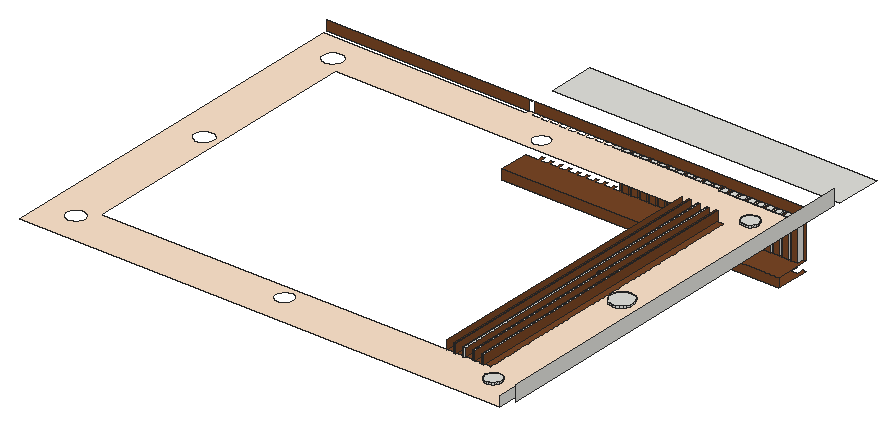
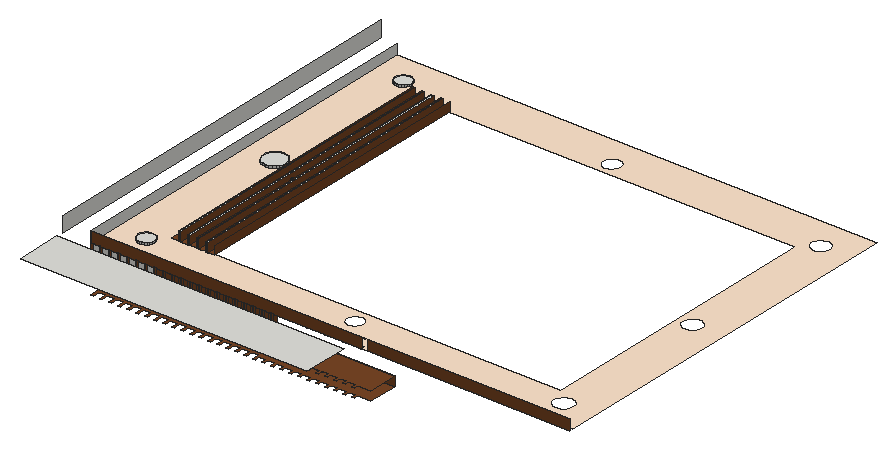
# SketchUp Ruby script. Lengths in inches.
U = 1.inch
M = Sketchup.active_model
def pt(a) = Geom::Point3d.new(a.map { |v| v * U })
def face(e, loops, mat)
  f = e.add_face(loops[0].map { |a| pt(a) })
  loops[1..].each { |l| e.add_face(l.map { |a| pt(a) }).erase! }
  f.material = f.back_material = mat if mat
  f
end
# faces: each face lists its corners as indices into pts; further lists are holes
def faces(e, pts, list, mat = nil) = list.each { |f| face(e, (f[0].is_a?(Array) ? f : [f]).map { |l| l.map { |i| pts[i] } }, mat) }
# xy, xz, yz: faces in a plane at the given z, y or x. An outline is a flat list of corners, or four numbers for a rectangle; further outlines are holes
def ring(l) = l.size == 4 ? [[l[0], l[1]], [l[2], l[1]], [l[2], l[3]], [l[0], l[3]]] : l.each_slice(2).to_a
def flat(e, list, mat, &to3) = list.each { |f| face(e, (f[0].is_a?(Array) ? f : [f]).map { |l| ring(l).map { |u, v| to3.(u, v) } }, mat) }
def xy(e, z, list, mat = nil) = flat(e, list, mat) { |x, y| [x, y, z] }
def xz(e, y, list, mat = nil) = flat(e, list, mat) { |x, z| [x, y, z] }
def yz(e, x, list, mat = nil) = flat(e, list, mat) { |y, z| [x, y, z] }
def lines(e, pts, list) = list.each { |a, b| e.add_line(pt(pts[a]), pt(pts[b])) }
# prism: a flat outline (further loops are holes) pulled along v
def prism(e, loops, v, mat = nil)
  f = face(e, loops, mat); d = Geom::Vector3d.new(v.map { |x| x * U })
  f.pushpull(f.normal.samedirection?(d) ? d.length : -d.length)
end
def box(e, o, s, mat = nil) = prism(e, [[o, [o[0] + s[0], o[1], o[2]], [o[0] + s[0], o[1] + s[1], o[2]], [o[0], o[1] + s[1], o[2]]]], [0, 0, s[2]], mat)
def at(x, y, z, deg = 0) = Geom::Transformation.translation(pt([x, y, z])) * Geom::Transformation.rotation(ORIGIN, Z_AXIS, deg.degrees)
def axes(o, x, y, z) = Geom::Transformation.new([*x, 0, *y, 0, *z, 0, *pt(o).to_a, 1])
def part(name) = M.definitions.add(name)
# library, detail: a bought-in or finely detailed component or shape, given as its bounding box
def library(name, o, s) = part(name).tap { |d| box(d.entities, o, s) }
def detail(e, o, s) = box(e.add_group.entities, o, s)
def put(e, d, t, mat = nil) = e.add_instance(d, t).tap { |i| i.material = mat if mat }
def group(e, t, mat = nil) = e.add_group.tap { |g| g.transformation = t; g.material = mat if mat }.entities
root = M.entities
M.materials.add("[Color C01]").color = [255, 229, 204]
M.materials.add("[Wood Veneer 01]").color = [120, 70, 37]
xy(root,101.64,[[[84.82,135.46,84.82,147.02,89.8,147.02,89.8,148.71,90.74,148.71,90.74,147.02,93.3,147.02,93.3,148.71,94.24,148.71,94.24,147.02,96.8,147.02,96.8,148.71,97.74,148.71,97.74,147.02,100.3,147.02,100.3,148.71,101.24,148.71,101.24,147.02,103.8,147.02,103.8,148.71,104.74,148.71,104.74,147.02,107.3,147.02,107.3,148.71,108.24,148.71,108.24,147.02,110.8,147.02,110.8,148.71,111.74,148.71,111.74,147.02,114.3,147.02,114.3,148.71,115.24,148.71,115.24,147.02,117.8,147.02,117.8,148.71,118.74,148.71,118.74,147.02,121.3,147.02,121.3,148.71,122.24,148.71,122.24,147.02,124.8,147.02,124.8,148.71,125.74,148.71,125.74,147.02,128.3,147.02,128.3,148.71,129.24,148.71,129.24,146.15,131.8,146.15,131.8,148.71,132.74,148.71,132.74,146.15,135.3,146.15,135.3,148.71,136.24,148.71,136.24,146.15,138.8,146.15,138.8,148.71,139.74,148.71,139.74,146.15,142.3,146.15,142.3,148.71,143.24,148.71,143.24,146.15,145.8,146.15,145.8,148.71,146.74,148.71,146.74,146.15,149.3,146.15,149.3,148.71,150.24,148.71,150.24,146.15,152.8,146.15,152.8,148.71,153.74,148.71,153.74,146.15,156.3,146.15,156.3,148.71,157.24,148.71,157.24,146.15,159.8,146.15,159.8,148.71,160.74,148.71,160.74,146.15,163.3,146.15,163.3,148.71,164.24,148.71,164.24,146.15,166.8,146.15,166.8,148.71,167.74,148.71,167.74,146.15,170.3,146.15,170.3,148.71,171.24,148.71,171.24,146.15,173.8,146.15,173.8,148.71,174.74,148.71,174.74,146.15,177.3,146.15,177.3,148.71,178.24,148.71,178.24,146.15,180.8,146.15,180.8,148.71,181.74,148.71,181.74,146.15,184.3,146.15,184.3,148.71,185.24,148.71,185.24,146.15,187.8,146.15,187.8,148.71,188.74,148.71,188.74,146.15,191.3,146.15,191.3,148.71,192.34,148.71,192.34,135.46],[148.54,139.05,149.09,139.12,149.6,139.33,150.04,139.67,150.38,140.11,150.59,140.625,150.66,141.17,150.59,141.72,150.38,142.24,150.04,142.68,149.6,143.01,149.09,143.23,148.54,143.3,147.99,143.23,147.48,143.01,147.04,142.68,146.7,142.24,146.49,141.72,146.41,141.17,146.49,140.625,146.7,140.11,147.04,139.67,147.48,139.33,147.99,139.12],[184.41,139.05,184.96,139.12,185.48,139.33,185.92,139.67,186.25,140.11,186.47,140.625,186.54,141.17,186.47,141.72,186.25,142.24,185.92,142.68,185.48,143.01,184.96,143.23,184.41,143.3,183.86,143.23,183.35,143.01,182.91,142.68,182.57,142.24,182.36,141.72,182.29,141.17,182.36,140.625,182.57,140.11,182.91,139.67,183.35,139.33,183.86,139.12],[108.65,138.59,109.2,138.66,109.71,138.87,110.15,139.21,110.49,139.65,110.7,140.16,110.77,140.71,110.7,141.26,110.49,141.77,110.15,142.21,109.71,142.55,109.2,142.76,108.65,142.84,108.1,142.76,107.59,142.55,107.15,142.21,106.81,141.77,106.6,141.26,106.52,140.71,106.6,140.16,106.81,139.65,107.15,139.21,107.59,138.87,108.1,138.66]]],"[Wood Veneer 01]")
xy(root,102.39,[[148.54,139.05,147.99,139.12,147.48,139.33,147.04,139.67,146.7,140.11,146.49,140.625,146.41,141.17,146.49,141.72,146.7,142.24,147.04,142.68,147.48,143.01,147.99,143.23,148.54,143.3,149.09,143.23,149.6,143.01,150.04,142.68,150.38,142.24,150.59,141.72,150.66,141.17,150.59,140.625,150.38,140.11,150.04,139.67,149.6,139.33,149.09,139.12],[184.41,139.05,183.86,139.12,183.35,139.33,182.91,139.67,182.57,140.11,182.36,140.625,182.29,141.17,182.36,141.72,182.57,142.24,182.91,142.68,183.35,143.01,183.86,143.23,184.41,143.3,184.96,143.23,185.48,143.01,185.92,142.68,186.25,142.24,186.47,141.72,186.54,141.17,186.47,140.625,186.25,140.11,185.92,139.67,185.48,139.33,184.96,139.12]])
xy(root,105.33,[[84.82,135.46,192.34,135.46,192.34,148.71,191.3,148.71,191.3,146.15,188.74,146.15,188.74,148.71,187.8,148.71,187.8,146.15,185.24,146.15,185.24,148.71,184.3,148.71,184.3,146.15,181.74,146.15,181.74,148.71,180.8,148.71,180.8,146.15,178.24,146.15,178.24,148.71,177.3,148.71,177.3,146.15,174.74,146.15,174.74,148.71,173.8,148.71,173.8,146.15,171.24,146.15,171.24,148.71,170.3,148.71,170.3,146.15,167.74,146.15,167.74,148.71,166.8,148.71,166.8,146.15,164.24,146.15,164.24,148.71,163.3,148.71,163.3,146.15,160.74,146.15,160.74,148.71,159.8,148.71,159.8,147.02,157.24,147.02,157.24,148.71,156.3,148.71,156.3,147.02,153.74,147.02,153.74,148.71,152.8,148.71,152.8,147.02,150.24,147.02,150.24,148.71,149.3,148.71,149.3,147.02,146.74,147.02,146.74,148.71,145.8,148.71,145.8,147.02,143.24,147.02,143.24,148.71,142.3,148.71,142.3,147.02,139.74,147.02,139.74,148.71,138.8,148.71,138.8,147.02,136.24,147.02,136.24,148.71,135.3,148.71,135.3,147.02,132.74,147.02,132.74,148.71,131.8,148.71,131.8,147.02,129.24,147.02,129.24,148.71,128.3,148.71,128.3,147.02,125.74,147.02,125.74,148.71,124.8,148.71,124.8,147.02,122.24,147.02,122.24,148.71,121.3,148.71,121.3,147.02,118.74,147.02,118.74,148.71,117.8,148.71,117.8,147.02,115.24,147.02,115.24,148.71,114.3,148.71,114.3,147.02,111.74,147.02,111.74,148.71,110.8,148.71,110.8,147.02,108.24,147.02,108.24,148.71,107.3,148.71,107.3,147.02,104.74,147.02,104.74,148.71,103.8,148.71,103.8,147.02,101.24,147.02,101.24,148.71,100.3,148.71,100.3,147.02,97.74,147.02,97.74,148.71,96.8,148.71,96.8,147.02,94.24,147.02,94.24,148.71,93.3,148.71,93.3,147.02,90.74,147.02,90.74,148.71,89.8,148.71,89.8,147.02,84.82,147.02]],"[Wood Veneer 01]")
xy(root,119.8125,[[160.74,146.15,163.3,148.71],[164.24,146.15,166.8,148.71],[167.74,146.15,170.3,148.71],[171.24,146.15,173.8,148.71],[174.74,146.15,177.3,148.71],
  [178.24,146.15,180.8,148.71],[181.74,146.15,184.3,148.71],[185.24,146.15,187.8,148.71],[188.74,146.15,191.3,148.71],[118.74,147.02,121.3,148.71],
  [122.24,147.02,124.8,148.71],[125.74,147.02,128.3,148.71],[129.24,147.02,131.8,148.71],[132.74,147.02,135.3,148.71],[136.24,147.02,138.8,148.71],
  [139.74,147.02,142.3,148.71],[143.24,147.02,145.8,148.71],[146.74,147.02,149.3,148.71],[150.24,147.02,152.8,148.71],[153.74,147.02,156.3,148.71],
  [157.24,147.02,159.8,148.71]])
xy(root,119.8125,[[[6.1,0,6.1,147.26,84.82,147.26,84.82,148.71,87.24,148.71,87.24,147.02,89.8,147.02,89.8,148.71,90.74,148.71,90.74,147.02,93.3,147.02,93.3,148.71,94.24,148.71,94.24,147.02,96.8,147.02,96.8,148.71,97.74,148.71,97.74,147.02,100.3,147.02,100.3,148.71,101.24,148.71,101.24,147.02,103.8,147.02,103.8,148.71,104.74,148.71,104.74,147.02,107.3,147.02,107.3,148.71,108.24,148.71,108.24,147.02,110.8,147.02,110.8,148.71,111.74,148.71,111.74,147.02,114.3,147.02,114.3,148.71,115.24,148.71,115.24,147.02,117.8,147.02,117.8,148.71,118.74,148.71,118.74,147.02,121.3,147.02,121.3,148.71,122.24,148.71,122.24,147.02,124.8,147.02,124.8,148.71,125.74,148.71,125.74,147.02,128.3,147.02,128.3,148.71,129.24,148.71,129.24,147.02,131.8,147.02,131.8,148.71,132.74,148.71,132.74,147.02,135.3,147.02,135.3,148.71,136.24,148.71,136.24,147.02,138.8,147.02,138.8,148.71,139.74,148.71,139.74,147.02,142.3,147.02,142.3,148.71,143.24,148.71,143.24,147.02,145.8,147.02,145.8,148.71,146.74,148.71,146.74,147.02,149.3,147.02,149.3,148.71,150.24,148.71,150.24,147.02,152.8,147.02,152.8,148.71,153.74,148.71,153.74,147.02,156.3,147.02,156.3,148.71,157.24,148.71,157.24,147.02,159.8,147.02,159.8,148.71,160.74,148.71,160.74,146.15,163.3,146.15,163.3,148.71,164.24,148.71,164.24,146.15,166.8,146.15,166.8,148.71,167.74,148.71,167.74,146.15,170.3,146.15,170.3,148.71,171.24,148.71,171.24,146.15,173.8,146.15,173.8,148.71,174.74,148.71,174.74,146.15,177.3,146.15,177.3,148.71,178.24,148.71,178.24,146.15,180.8,146.15,180.8,148.71,181.74,148.71,181.74,146.15,184.3,146.15,184.3,148.71,185.24,148.71,185.24,146.15,187.8,146.15,187.8,148.71,188.74,148.71,188.74,146.15,191.3,146.15,191.3,148.71,192.34,148.71,192.34,0],[23.52,17.41,174.92,131.3],[180.34,69.92,181.48,70.07,182.55,70.51,183.47,71.22,184.18,72.14,184.62,73.21,184.77,74.36,184.62,75.5,184.18,76.57,183.47,77.49,182.55,78.2,181.48,78.64,180.34,78.79,179.1875,78.64,178.12,78.2,177.2,77.49,176.49,76.57,176.05,75.5,175.9,74.36,176.05,73.21,176.49,72.14,177.2,71.22,178.12,70.51,179.1875,70.07],[18.1,132.84,19.11,132.97,20.04,133.35,20.84,133.97,21.46,134.77,21.85,135.71,21.98,136.71,21.85,137.71,21.46,138.65,20.84,139.45,20.04,140.07,19.11,140.45,18.1,140.59,17.1,140.45,16.16,140.07,15.36,139.45,14.75,138.65,14.36,137.71,14.23,136.71,14.36,135.71,14.75,134.77,15.36,133.97,16.16,133.35,17.1,132.97],[17.86,70.55,18.86,70.62,19.8,70.94,20.625,71.49,21.28,72.24,21.72,73.14,21.91,74.12,21.84,75.11,21.52,76.05,20.96,76.875,20.21,77.53,19.32,77.97,18.34,78.16,17.35,78.09,16.41,77.77,15.58,77.22,14.93,76.47,14.49,75.57,14.3,74.6,14.36,73.6,14.6875,72.66,15.24,71.83,15.99,71.18,16.89,70.74],[18.23,8.31,19.18,8.47,20.06,8.875,20.8,9.49,21.36,10.27,21.7,11.17,21.79,12.13,21.63,13.08,21.23,13.96,20.62,14.7,19.83,15.26,18.93,15.59,17.97,15.69,17.02,15.53,16.15,15.125,15.4,14.51,14.85,13.73,14.51,12.83,14.42,11.87,14.58,10.92,14.98,10.04,15.59,9.3,16.37,8.74,17.27,8.41],[99.22,8.5,100.125,8.62,100.97,8.97,101.69,9.53,102.25,10.25,102.6,11.09,102.72,12,102.6,12.91,102.25,13.75,101.69,14.47,100.97,15.03,100.125,15.38,99.22,15.5,98.3125,15.38,97.47,15.03,96.74,14.47,96.1875,13.75,95.84,12.91,95.72,12,95.84,11.09,96.1875,10.25,96.74,9.53,97.47,8.97,98.3125,8.62],[99.22,133.4,100.08,133.51,100.875,133.84,101.5625,134.37,102.09,135.05,102.42,135.85,102.53,136.71,102.42,137.57,102.09,138.37,101.5625,139.05,100.875,139.58,100.08,139.91,99.22,140.02,98.36,139.91,97.5625,139.58,96.875,139.05,96.35,138.37,96.02,137.57,95.91,136.71,96.02,135.85,96.35,135.05,96.875,134.37,97.5625,133.84,98.36,133.51],[180.34,133.46,181.18,133.57,181.96,133.9,182.63,134.41,183.15,135.09,183.47,135.87,183.59,136.71,183.47,137.55,183.15,138.34,182.63,139.01,181.96,139.52,181.18,139.85,180.34,139.96,179.49,139.85,178.71,139.52,178.04,139.01,177.52,138.34,177.2,137.55,177.09,136.71,177.2,135.87,177.52,135.09,178.04,134.41,178.71,133.9,179.49,133.57],[180.34,8.8125,181.16,8.92,181.93,9.24,182.59,9.75,183.1,10.41,183.41,11.18,183.52,12,183.41,12.82,183.1,13.59,182.59,14.25,181.93,14.76,181.16,15.08,180.34,15.1875,179.51,15.08,178.74,14.76,178.08,14.25,177.57,13.59,177.26,12.82,177.15,12,177.26,11.18,177.57,10.41,178.08,9.75,178.74,9.24,179.51,8.92]]],"[Color C01]")
xy(root,119.8125,[[157.97,17.41,160.67,131.3],[161.53,17.41,164.23,131.3],[[165.09,17.41,167.8,131.3],[166.45,80.57,166.77,80.63,167.0625,80.77,167.3125,80.98,167.5,81.25,167.61,81.56,167.64,81.88,167.58,82.2,167.44,82.5,167.23,82.75,166.96,82.93,166.66,83.04,166.33,83.07,166.01,83.01,165.71,82.875,165.46,82.66,165.28,82.4,165.17,82.09,165.14,81.76,165.2,81.44,165.34,81.15,165.55,80.9,165.82,80.71,166.12,80.6]],[168.65,17.41,171.36,131.3],[172.22,17.41,174.92,131.3]],"[Wood Veneer 01]")
xy(root,120.5,[[180.34,8.8125,179.51,8.92,178.74,9.24,178.08,9.75,177.57,10.41,177.26,11.18,177.15,12,177.26,12.82,177.57,13.59,178.08,14.25,178.74,14.76,179.51,15.08,180.34,15.1875,181.16,15.08,181.93,14.76,182.59,14.25,183.1,13.59,183.41,12.82,183.52,12,183.41,11.18,183.1,10.41,182.59,9.75,181.93,9.24,181.16,8.92],[180.34,69.92,179.1875,70.07,178.12,70.51,177.2,71.22,176.49,72.14,176.05,73.21,175.9,74.36,176.05,75.5,176.49,76.57,177.2,77.49,178.12,78.2,179.1875,78.64,180.34,78.79,181.48,78.64,182.55,78.2,183.47,77.49,184.18,76.57,184.62,75.5,184.77,74.36,184.62,73.21,184.18,72.14,183.47,71.22,182.55,70.51,181.48,70.07],[180.34,133.46,179.49,133.57,178.71,133.9,178.04,134.41,177.52,135.09,177.2,135.87,177.09,136.71,177.2,137.55,177.52,138.34,178.04,139.01,178.71,139.52,179.49,139.85,180.34,139.96,181.18,139.85,181.96,139.52,182.63,139.01,183.15,138.34,183.47,137.55,183.59,136.71,183.47,135.87,183.15,135.09,182.63,134.41,181.96,133.9,181.18,133.57]])
xy(root,121.5,[[166.45,80.57,166.12,80.6,165.82,80.71,165.55,80.9,165.34,81.15,165.2,81.44,165.14,81.76,165.17,82.09,165.28,82.4,165.46,82.66,165.71,82.875,166.01,83.01,166.33,83.07,166.66,83.04,166.96,82.93,167.23,82.75,167.44,82.5,167.58,82.2,167.64,81.88,167.61,81.56,167.5,81.25,167.3125,80.98,167.0625,80.77,166.77,80.63]])
xy(root,123.25,[[160.67,17.41,161.53,131.3],[164.23,17.41,165.09,131.3],[167.8,17.41,168.65,131.3],[171.36,17.41,172.22,131.3]])
xy(root,123.71,[[87.07,157.4375,198.4375,175.3125]])
xz(root,17.41,[[160.67,119.8125,161.53,123.25],[164.23,119.8125,165.09,123.25],[167.8,119.8125,168.65,123.25],[171.36,119.8125,172.22,123.25]])
xz(root,131.3,[[160.67,119.8125,161.53,123.25],[164.23,119.8125,165.09,123.25],[167.8,119.8125,168.65,123.25],[171.36,119.8125,172.22,123.25]])
xz(root,135.46,[[84.82,101.64,192.34,105.33]],"[Wood Veneer 01]")
xz(root,146.15,[[160.74,105.33,163.3,119.8125],[164.24,105.33,166.8,119.8125],[167.74,105.33,170.3,119.8125],[171.24,105.33,173.8,119.8125],[174.74,105.33,177.3,119.8125],
  [178.24,105.33,180.8,119.8125],[181.74,105.33,184.3,119.8125],[185.24,105.33,187.8,119.8125],[188.74,105.33,191.3,119.8125]],"[Wood Veneer 01]")
xz(root,147.02,[[122.24,105.33,124.8,119.8125],[125.74,105.33,128.3,119.8125],[129.24,105.33,131.8,119.8125],[132.74,105.33,135.3,119.8125],[136.24,105.33,138.8,119.8125],
  [139.74,105.33,142.3,119.8125],[143.24,105.33,145.8,119.8125],[146.74,105.33,149.3,119.8125],[150.24,105.33,152.8,119.8125],[153.74,105.33,156.3,119.8125],
  [157.24,105.33,159.8,119.8125]],"[Wood Veneer 01]")
xz(root,148.71,[[121.3,105.33,122.24,119.8125],[124.8,105.33,125.74,119.8125],[128.3,105.33,129.24,119.8125],[131.8,105.33,132.74,119.8125],[135.3,105.33,136.24,119.8125],
  [138.8,105.33,139.74,119.8125],[142.3,105.33,143.24,119.8125],[145.8,105.33,146.74,119.8125],[149.3,105.33,150.24,119.8125],[152.8,105.33,153.74,119.8125],
  [156.3,105.33,157.24,119.8125],[159.8,105.33,160.74,119.8125],[163.3,105.33,164.24,119.8125],[166.8,105.33,167.74,119.8125],[170.3,105.33,171.24,119.8125],
  [173.8,105.33,174.74,119.8125],[177.3,105.33,178.24,119.8125],[180.8,105.33,181.74,119.8125],[184.3,105.33,185.24,119.8125],[187.8,105.33,188.74,119.8125],
  [191.3,105.33,192.34,119.8125],[6.1,119.8125,84.82,119.8125,84.82,123.71,87.07,123.71,87.07,119.8125,192.34,119.8125,192.34,123.75,6.1,123.75]],"[Wood Veneer 01]")
yz(root,121.3,[[147.02,105.33,148.71,119.8125]],"[Wood Veneer 01]")
yz(root,122.24,[[147.02,105.33,148.71,119.8125]])
yz(root,124.8,[[147.02,105.33,148.71,119.8125]],"[Wood Veneer 01]")
yz(root,125.74,[[147.02,105.33,148.71,119.8125]])
yz(root,128.3,[[147.02,105.33,148.71,119.8125]],"[Wood Veneer 01]")
yz(root,129.24,[[147.02,105.33,148.71,119.8125]])
yz(root,131.8,[[147.02,105.33,148.71,119.8125]],"[Wood Veneer 01]")
yz(root,132.74,[[147.02,105.33,148.71,119.8125]],"[Wood Veneer 01]")
yz(root,135.3,[[147.02,105.33,148.71,119.8125]],"[Wood Veneer 01]")
yz(root,136.24,[[147.02,105.33,148.71,119.8125]],"[Wood Veneer 01]")
yz(root,138.8,[[147.02,105.33,148.71,119.8125]],"[Wood Veneer 01]")
yz(root,139.74,[[147.02,105.33,148.71,119.8125]],"[Wood Veneer 01]")
yz(root,142.3,[[147.02,105.33,148.71,119.8125]],"[Wood Veneer 01]")
yz(root,143.24,[[147.02,105.33,148.71,119.8125]],"[Wood Veneer 01]")
yz(root,145.8,[[147.02,105.33,148.71,119.8125]],"[Wood Veneer 01]")
yz(root,146.74,[[147.02,105.33,148.71,119.8125]],"[Wood Veneer 01]")
yz(root,149.3,[[147.02,105.33,148.71,119.8125]],"[Wood Veneer 01]")
yz(root,150.24,[[147.02,105.33,148.71,119.8125]],"[Wood Veneer 01]")
yz(root,152.8,[[147.02,105.33,148.71,119.8125]],"[Wood Veneer 01]")
yz(root,153.74,[[147.02,105.33,148.71,119.8125]],"[Wood Veneer 01]")
yz(root,156.3,[[147.02,105.33,148.71,119.8125]],"[Wood Veneer 01]")
yz(root,157.24,[[147.02,105.33,148.71,119.8125]],"[Wood Veneer 01]")
yz(root,157.97,[[17.41,119.8125,131.3,123.25]],"[Wood Veneer 01]")
yz(root,159.8,[[147.02,105.33,148.71,119.8125]],"[Wood Veneer 01]")
yz(root,160.67,[[17.41,119.8125,131.3,123.25]],"[Wood Veneer 01]")
yz(root,160.74,[[146.15,105.33,148.71,119.8125]],"[Wood Veneer 01]")
yz(root,161.53,[[17.41,119.8125,131.3,123.25]],"[Wood Veneer 01]")
yz(root,163.3,[[146.15,105.33,148.71,119.8125]],"[Wood Veneer 01]")
yz(root,164.23,[[17.41,119.8125,131.3,123.25]],"[Wood Veneer 01]")
yz(root,164.24,[[146.15,105.33,148.71,119.8125]],"[Wood Veneer 01]")
yz(root,165.09,[[17.41,119.8125,131.3,123.25]],"[Wood Veneer 01]")
yz(root,166.8,[[146.15,105.33,148.71,119.8125]],"[Wood Veneer 01]")
yz(root,167.74,[[146.15,105.33,148.71,119.8125]],"[Wood Veneer 01]")
yz(root,167.8,[[17.41,119.8125,131.3,123.25]],"[Wood Veneer 01]")
yz(root,168.65,[[17.41,119.8125,131.3,123.25]],"[Wood Veneer 01]")
yz(root,170.3,[[146.15,105.33,148.71,119.8125]])
yz(root,171.24,[[146.15,105.33,148.71,119.8125]],"[Wood Veneer 01]")
yz(root,171.36,[[17.41,119.8125,131.3,123.25]],"[Wood Veneer 01]")
yz(root,172.22,[[17.41,119.8125,131.3,123.25]],"[Wood Veneer 01]")
yz(root,173.8,[[146.15,105.33,148.71,119.8125]])
yz(root,174.74,[[146.15,105.33,148.71,119.8125]],"[Wood Veneer 01]")
yz(root,177.3,[[146.15,105.33,148.71,119.8125]])
yz(root,178.24,[[146.15,105.33,148.71,119.8125]],"[Wood Veneer 01]")
yz(root,180.8,[[146.15,105.33,148.71,119.8125]])
yz(root,181.74,[[146.15,105.33,148.71,119.8125]],"[Wood Veneer 01]")
yz(root,184.3,[[146.15,105.33,148.71,119.8125]])
yz(root,185.24,[[146.15,105.33,148.71,119.8125]],"[Wood Veneer 01]")
yz(root,187.8,[[146.15,105.33,148.71,119.8125]])
yz(root,188.74,[[146.15,105.33,148.71,119.8125]],"[Wood Veneer 01]")
yz(root,191.3,[[146.15,105.33,148.71,119.8125]])
yz(root,192.34,[[0,119.8125,148.71,123.75]])
yz(root,198.4375,[[0,123.75,154.8125,129.75]])
p = [[148.54,139.05,101.64],[147.99,139.12,101.64],[147.99,139.12,102.39],[148.54,139.05,102.39],[149.09,139.12,101.64],[149.09,139.12,102.39],
  [184.41,139.05,101.64],[183.86,139.12,101.64],[183.86,139.12,102.39],[184.41,139.05,102.39],[184.96,139.12,101.64],[184.96,139.12,102.39],
  [147.48,139.33,101.64],[147.48,139.33,102.39],[149.6,139.33,101.64],[149.6,139.33,102.39],[183.35,139.33,101.64],[183.35,139.33,102.39],
  [185.48,139.33,101.64],[185.48,139.33,102.39],[147.04,139.67,101.64],[147.04,139.67,102.39],[150.04,139.67,101.64],[150.04,139.67,102.39],
  [182.91,139.67,101.64],[182.91,139.67,102.39],[185.92,139.67,101.64],[185.92,139.67,102.39],[146.7,140.11,101.64],[146.7,140.11,102.39],
  [150.38,140.11,101.64],[150.38,140.11,102.39],[182.57,140.11,101.64],[182.57,140.11,102.39],[186.25,140.11,101.64],[186.25,140.11,102.39],
  [146.49,140.625,101.64],[146.49,140.625,102.39],[150.59,140.625,101.64],[150.59,140.625,102.39],[182.36,140.625,101.64],[182.36,140.625,102.39],
  [186.47,140.625,101.64],[186.47,140.625,102.39],[146.41,141.17,101.64],[146.41,141.17,102.39],[150.66,141.17,101.64],[150.66,141.17,102.39],
  [182.29,141.17,101.64],[182.29,141.17,102.39],[186.54,141.17,101.64],[186.54,141.17,102.39],[146.49,141.72,101.64],[146.49,141.72,102.39],
  [150.59,141.72,101.64],[150.59,141.72,102.39],[182.36,141.72,101.64],[182.36,141.72,102.39],[186.47,141.72,101.64],[186.47,141.72,102.39],
  [146.7,142.24,101.64],[146.7,142.24,102.39],[150.38,142.24,101.64],[150.38,142.24,102.39],[182.57,142.24,101.64],[182.57,142.24,102.39],
  [186.25,142.24,101.64],[186.25,142.24,102.39],[147.04,142.68,101.64],[147.04,142.68,102.39],[150.04,142.68,101.64],[150.04,142.68,102.39],
  [182.91,142.68,101.64],[182.91,142.68,102.39],[185.92,142.68,101.64],[185.92,142.68,102.39],[147.48,143.01,101.64],[147.48,143.01,102.39],
  [149.6,143.01,101.64],[149.6,143.01,102.39],[183.35,143.01,101.64],[183.35,143.01,102.39],[185.48,143.01,101.64],[185.48,143.01,102.39],
  [147.99,143.23,101.64],[147.99,143.23,102.39],[149.09,143.23,101.64],[149.09,143.23,102.39],[183.86,143.23,101.64],[183.86,143.23,102.39],
  [184.96,143.23,101.64],[184.96,143.23,102.39],[148.54,143.3,101.64],[148.54,143.3,102.39],[184.41,143.3,101.64],[184.41,143.3,102.39],
  [180.34,8.8125,119.8125],[179.51,8.92,119.8125],[179.51,8.92,120.5],[180.34,8.8125,120.5],[181.16,8.92,119.8125],[181.16,8.92,120.5],
  [178.74,9.24,119.8125],[178.74,9.24,120.5],[181.93,9.24,119.8125],[181.93,9.24,120.5],[178.08,9.75,119.8125],[178.08,9.75,120.5],
  [182.59,9.75,119.8125],[182.59,9.75,120.5],[177.57,10.41,119.8125],[177.57,10.41,120.5],[183.1,10.41,119.8125],[183.1,10.41,120.5],
  [177.26,11.18,119.8125],[177.26,11.18,120.5],[183.41,11.18,119.8125],[183.41,11.18,120.5],[177.15,12,119.8125],[177.15,12,120.5],
  [183.52,12,119.8125],[183.52,12,120.5],[177.26,12.82,119.8125],[177.26,12.82,120.5],[183.41,12.82,119.8125],[183.41,12.82,120.5],
  [177.57,13.59,119.8125],[177.57,13.59,120.5],[183.1,13.59,119.8125],[183.1,13.59,120.5],[178.08,14.25,119.8125],[178.08,14.25,120.5],
  [182.59,14.25,119.8125],[182.59,14.25,120.5],[178.74,14.76,119.8125],[178.74,14.76,120.5],[181.93,14.76,119.8125],[181.93,14.76,120.5],
  [179.51,15.08,119.8125],[179.51,15.08,120.5],[181.16,15.08,119.8125],[181.16,15.08,120.5],[180.34,15.1875,119.8125],[180.34,15.1875,120.5],
  [180.34,69.92,119.8125],[179.1875,70.07,119.8125],[179.1875,70.07,120.5],[180.34,69.92,120.5],[181.48,70.07,119.8125],[181.48,70.07,120.5],
  [178.12,70.51,119.8125],[178.12,70.51,120.5],[182.55,70.51,119.8125],[182.55,70.51,120.5],[177.2,71.22,119.8125],[177.2,71.22,120.5],
  [183.47,71.22,119.8125],[183.47,71.22,120.5],[176.49,72.14,119.8125],[176.49,72.14,120.5],[184.18,72.14,119.8125],[184.18,72.14,120.5],
  [176.05,73.21,119.8125],[176.05,73.21,120.5],[184.62,73.21,119.8125],[184.62,73.21,120.5],[175.9,74.36,119.8125],[175.9,74.36,120.5],
  [184.77,74.36,119.8125],[184.77,74.36,120.5],[176.05,75.5,119.8125],[176.05,75.5,120.5],[184.62,75.5,119.8125],[184.62,75.5,120.5],
  [176.49,76.57,119.8125],[176.49,76.57,120.5],[184.18,76.57,119.8125],[184.18,76.57,120.5],[177.2,77.49,119.8125],[177.2,77.49,120.5],
  [183.47,77.49,119.8125],[183.47,77.49,120.5],[178.12,78.2,119.8125],[178.12,78.2,120.5],[182.55,78.2,119.8125],[182.55,78.2,120.5],
  [179.1875,78.64,119.8125],[179.1875,78.64,120.5],[181.48,78.64,119.8125],[181.48,78.64,120.5],[180.34,78.79,119.8125],[180.34,78.79,120.5],
  [166.12,80.6,119.8125],[165.82,80.71,119.8125],[165.82,80.71,121.5],[166.12,80.6,121.5],[166.45,80.57,119.8125],[166.45,80.57,121.5],
  [166.77,80.63,119.8125],[166.77,80.63,121.5],[167.0625,80.77,119.8125],[167.0625,80.77,121.5],[165.55,80.9,119.8125],[165.55,80.9,121.5],
  [167.3125,80.98,119.8125],[167.3125,80.98,121.5],[165.34,81.15,119.8125],[165.34,81.15,121.5],[167.5,81.25,119.8125],[167.5,81.25,121.5],
  [165.2,81.44,119.8125],[165.2,81.44,121.5],[167.61,81.56,119.8125],[167.61,81.56,121.5],[165.14,81.76,119.8125],[165.14,81.76,121.5],
  [167.64,81.88,119.8125],[167.64,81.88,121.5],[165.17,82.09,119.8125],[165.17,82.09,121.5],[167.58,82.2,119.8125],[167.58,82.2,121.5],
  [165.28,82.4,119.8125],[165.28,82.4,121.5],[167.44,82.5,119.8125],[167.44,82.5,121.5],[165.46,82.66,119.8125],[165.46,82.66,121.5],
  [167.23,82.75,119.8125],[167.23,82.75,121.5],[165.71,82.875,119.8125],[165.71,82.875,121.5],[166.96,82.93,119.8125],[166.96,82.93,121.5],
  [166.01,83.01,119.8125],[166.01,83.01,121.5],[166.66,83.04,119.8125],[166.66,83.04,121.5],[166.33,83.07,119.8125],[166.33,83.07,121.5],
  [180.34,133.46,119.8125],[179.49,133.57,119.8125],[179.49,133.57,120.5],[180.34,133.46,120.5],[181.18,133.57,119.8125],[181.18,133.57,120.5],
  [178.71,133.9,119.8125],[178.71,133.9,120.5],[181.96,133.9,119.8125],[181.96,133.9,120.5],[178.04,134.41,119.8125],[178.04,134.41,120.5],
  [182.63,134.41,119.8125],[182.63,134.41,120.5],[177.52,135.09,119.8125],[177.52,135.09,120.5],[183.15,135.09,119.8125],[183.15,135.09,120.5],
  [177.2,135.87,119.8125],[177.2,135.87,120.5],[183.47,135.87,119.8125],[183.47,135.87,120.5],[177.09,136.71,119.8125],[177.09,136.71,120.5],
  [183.59,136.71,119.8125],[183.59,136.71,120.5],[177.2,137.55,119.8125],[177.2,137.55,120.5],[183.47,137.55,119.8125],[183.47,137.55,120.5],
  [177.52,138.34,119.8125],[177.52,138.34,120.5],[183.15,138.34,119.8125],[183.15,138.34,120.5],[178.04,139.01,119.8125],[178.04,139.01,120.5],
  [182.63,139.01,119.8125],[182.63,139.01,120.5],[178.71,139.52,119.8125],[178.71,139.52,120.5],[181.96,139.52,119.8125],[181.96,139.52,120.5],
  [179.49,139.85,119.8125],[179.49,139.85,120.5],[181.18,139.85,119.8125],[181.18,139.85,120.5],[180.34,139.96,119.8125],[180.34,139.96,120.5]]
faces(root,p,[[0,1,2,3],[4,0,3,5],[6,7,8,9],[10,6,9,11],[1,12,13,2],[14,4,5,15],[7,16,17,8],[18,10,11,19],
  [12,20,21,13],[22,14,15,23],[16,24,25,17],[26,18,19,27],[20,28,29,21],[30,22,23,31],[24,32,33,25],[34,26,27,35],
  [28,36,37,29],[38,30,31,39],[32,40,41,33],[42,34,35,43],[36,44,45,37],[46,38,39,47],[40,48,49,41],[50,42,43,51],
  [44,52,53,45],[54,46,47,55],[48,56,57,49],[58,50,51,59],[52,60,61,53],[62,54,55,63],[56,64,65,57],[66,58,59,67],
  [60,68,69,61],[70,62,63,71],[64,72,73,65],[74,66,67,75],[68,76,77,69],[78,70,71,79],[72,80,81,73],[82,74,75,83],
  [76,84,85,77],[86,78,79,87],[80,88,89,81],[90,82,83,91],[84,92,93,85],[92,86,87,93],[88,94,95,89],[94,90,91,95],
  [96,97,98,99],[100,96,99,101],[97,102,103,98],[104,100,101,105],[102,106,107,103],[108,104,105,109],[106,110,111,107],[112,108,109,113],
  [110,114,115,111],[116,112,113,117],[114,118,119,115],[120,116,117,121],[118,122,123,119],[124,120,121,125],[122,126,127,123],[128,124,125,129],
  [126,130,131,127],[132,128,129,133],[130,134,135,131],[136,132,133,137],[134,138,139,135],[140,136,137,141],[138,142,143,139],[142,140,141,143],
  [144,145,146,147],[148,144,147,149],[145,150,151,146],[152,148,149,153],[150,154,155,151],[156,152,153,157],[154,158,159,155],[160,156,157,161],
  [158,162,163,159],[164,160,161,165],[162,166,167,163],[168,164,165,169],[166,170,171,167],[172,168,169,173],[170,174,175,171],[176,172,173,177],
  [174,178,179,175],[180,176,177,181],[178,182,183,179],[184,180,181,185],[182,186,187,183],[188,184,185,189],[186,190,191,187],[190,188,189,191],
  [192,193,194,195],[196,192,195,197],[198,196,197,199],[200,198,199,201],[193,202,203,194],[204,200,201,205],[202,206,207,203],[208,204,205,209],
  [206,210,211,207],[212,208,209,213],[210,214,215,211],[216,212,213,217],[214,218,219,215],[220,216,217,221],[218,222,223,219],[224,220,221,225],
  [222,226,227,223],[228,224,225,229],[226,230,231,227],[232,228,229,233],[230,234,235,231],[236,232,233,237],[234,238,239,235],[238,236,237,239],
  [240,241,242,243],[244,240,243,245],[241,246,247,242],[248,244,245,249],[246,250,251,247],[252,248,249,253],[250,254,255,251],[256,252,253,257],
  [254,258,259,255],[260,256,257,261],[258,262,263,259],[264,260,261,265],[262,266,267,263],[268,264,265,269],[266,270,271,267],[272,268,269,273],
  [270,274,275,271],[276,272,273,277],[274,278,279,275],[280,276,277,281],[278,282,283,279],[284,280,281,285],[282,286,287,283],[286,284,285,287]])
